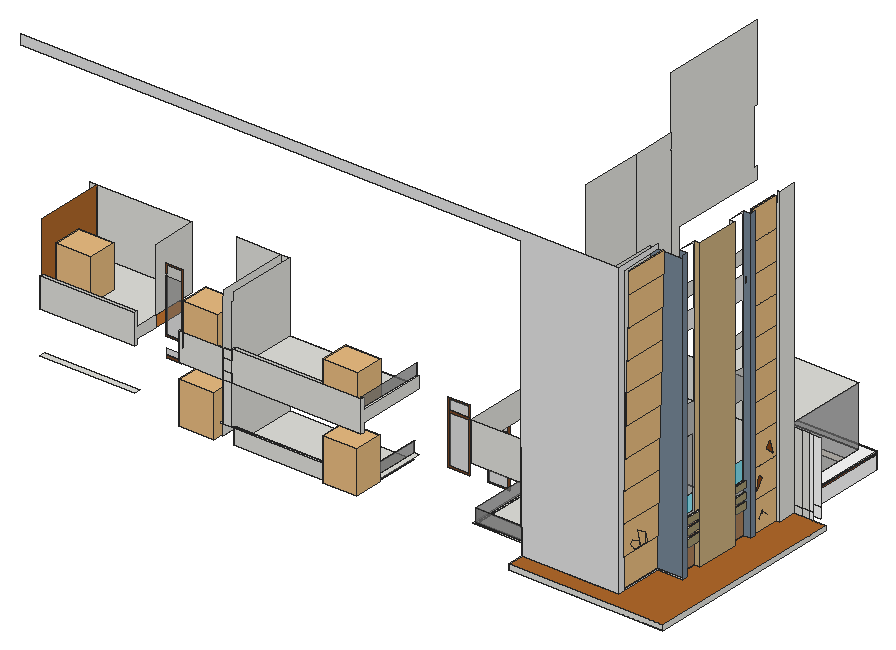
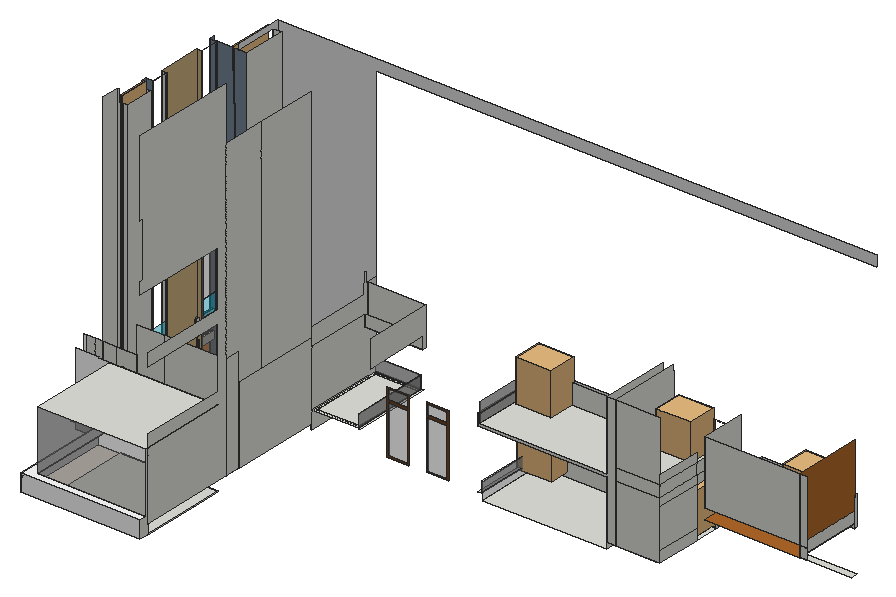
# SketchUp Ruby script. Lengths in inches.
U = 1.inch
M = Sketchup.active_model
def pt(a) = Geom::Point3d.new(a.map { |v| v * U })
def face(e, loops, mat)
  f = e.add_face(loops[0].map { |a| pt(a) })
  loops[1..].each { |l| e.add_face(l.map { |a| pt(a) }).erase! }
  f.material = f.back_material = mat if mat
  f
end
# faces: each face lists its corners as indices into pts; further lists are holes
def faces(e, pts, list, mat = nil) = list.each { |f| face(e, (f[0].is_a?(Array) ? f : [f]).map { |l| l.map { |i| pts[i] } }, mat) }
# xy, xz, yz: faces in a plane at the given z, y or x. An outline is a flat list of corners, or four numbers for a rectangle; further outlines are holes
def ring(l) = l.size == 4 ? [[l[0], l[1]], [l[2], l[1]], [l[2], l[3]], [l[0], l[3]]] : l.each_slice(2).to_a
def flat(e, list, mat, &to3) = list.each { |f| face(e, (f[0].is_a?(Array) ? f : [f]).map { |l| ring(l).map { |u, v| to3.(u, v) } }, mat) }
def xy(e, z, list, mat = nil) = flat(e, list, mat) { |x, y| [x, y, z] }
def xz(e, y, list, mat = nil) = flat(e, list, mat) { |x, z| [x, y, z] }
def yz(e, x, list, mat = nil) = flat(e, list, mat) { |y, z| [x, y, z] }
def lines(e, pts, list) = list.each { |a, b| e.add_line(pt(pts[a]), pt(pts[b])) }
# prism: a flat outline (further loops are holes) pulled along v
def prism(e, loops, v, mat = nil)
  f = face(e, loops, mat); d = Geom::Vector3d.new(v.map { |x| x * U })
  f.pushpull(f.normal.samedirection?(d) ? d.length : -d.length)
end
def box(e, o, s, mat = nil) = prism(e, [[o, [o[0] + s[0], o[1], o[2]], [o[0] + s[0], o[1] + s[1], o[2]], [o[0], o[1] + s[1], o[2]]]], [0, 0, s[2]], mat)
def at(x, y, z, deg = 0) = Geom::Transformation.translation(pt([x, y, z])) * Geom::Transformation.rotation(ORIGIN, Z_AXIS, deg.degrees)
def axes(o, x, y, z) = Geom::Transformation.new([*x, 0, *y, 0, *z, 0, *pt(o).to_a, 1])
def part(name) = M.definitions.add(name)
# library, detail: a bought-in or finely detailed component or shape, given as its bounding box
def library(name, o, s) = part(name).tap { |d| box(d.entities, o, s) }
def detail(e, o, s) = box(e.add_group.entities, o, s)
def put(e, d, t, mat = nil) = e.add_instance(d, t).tap { |i| i.material = mat if mat }
def group(e, t, mat = nil) = e.add_group.tap { |g| g.transformation = t; g.material = mat if mat }.entities
root = M.entities
M.materials.add("[0030_OldLace]").color = [253, 245, 230]
M.materials.add("[0042_Sienna]").color = [160, 82, 45]
M.materials.add("[0043_SaddleBrown]").color = [139, 69, 19]
M.materials.add("[0110_LightSlateGray]").color = [119, 136, 153]
M.materials.add("[0128_White]").color = [255, 255, 255]
M.materials.add("[0129_WhiteSmoke]").color = [245, 245, 245]
M.materials.add("[Polished Concrete Old]").color = [229, 229, 229]
M.materials.add("[Translucent Glass Gray]").color = [128, 128, 128]
M.materials["[Translucent Glass Gray]"].alpha = 0.5
M.materials.add("[Translucent Glass Tinted]").color = [8, 201, 241]
M.materials["[Translucent Glass Tinted]"].alpha = 0.48
M.materials.add("[Wood Bamboo]").color = [177, 105, 43]
M.materials.add("[Wood Floor Light]").color = [204, 176, 127]
M.materials.add("[Wood Floor]").color = [155, 105, 61]
M.materials.add("[Wood Lumber ButtJoined]").color = [164, 152, 112]
M.materials.add("[Wood Veneer 01]").color = [120, 70, 37]
c1 = library("Plant+(3)",[-15.5,2.64,0],[117.71,96.38,184.75])
c2 = library("Group\#2",[2.66,0,2.66],[81.3,1.18,61.61])
c3 = part("Decorative screen panels")
put(c3.entities,c2,axes([-6.34,-1.57,-2.66],[1.10721,0,0],[0,-0.19,0],[0,0,1]))
put(c3.entities,c2,axes([-6.34,0,59.33],[1.10721,0,0],[0,-0.19,0],[0,0,1]))
put(c3.entities,c2,axes([-6.34,1.57,121.32],[1.10721,0,0],[0,-0.19,0],[0,0,1]))
put(c3.entities,c2,axes([-6.34,3.15,183.3],[1.10721,0,0],[0,-0.19,0],[0,0,1]))
put(c3.entities,c2,axes([-6.34,4.72,245.29],[1.10721,0,0],[0,-0.19,0],[0,0,1]))
put(c3.entities,c2,axes([-6.34,6.3,307.28],[1.10721,0,0],[0,-0.19,0],[0,0,1]))
put(c3.entities,c2,axes([-6.34,7.875,369.27],[1.10721,0,0],[0,-0.19,0],[0,0,1]))
put(c3.entities,c2,axes([-6.34,9.45,431.25],[1.10721,0,0],[0,-0.19,0],[0,0,1]))
put(c3.entities,c2,axes([-6.34,11.02,493.24],[1.10721,0,0],[0,-0.19,0],[0,0,1]))
put(c3.entities,c2,axes([-6.34,10.61,555.97],[1.10721,0,0],[0,1.4896,0],[0,0,0.7225]))
put(c3.entities,c2,axes([-255.6,43,-5.47],[0.74066,0,0],[0,3.6727,0],[0,0,1]))
put(c3.entities,c2,axes([-255.6,43,55.32],[0.74066,0,0],[0,3.6727,0],[0,0,1]))
put(c3.entities,c2,axes([-255.6,43,116.1],[0.74066,0,0],[0,3.6727,0],[0,0,1]))
put(c3.entities,c2,axes([-255.6,43,176.89],[0.74066,0,0],[0,3.6727,0],[0,0,1]))
put(c3.entities,c2,axes([-255.6,43,237.68],[0.74066,0,0],[0,3.6727,0],[0,0,1]))
put(c3.entities,c2,axes([-255.6,43,298.47],[0.74066,0,0],[0,3.6727,0],[0,0,1]))
put(c3.entities,c2,axes([-255.6,43,359.26],[0.74066,0,0],[0,3.6727,0],[0,0,1]))
put(c3.entities,c2,axes([-255.6,43,420.05],[0.74066,0,0],[0,3.6727,0],[0,0,1]))
put(c3.entities,c2,axes([-255.6,43,480.84],[0.74066,0,0],[0,3.6727,0],[0,0,1]))
put(c3.entities,c2,axes([-255.6,43,543.4],[0.74066,0,0],[0,3.6727,0],[0,0,1]))
xy(root,140.13,[[1381.11,725.91,1632.4375,929.16]],"[0030_OldLace]")
xy(root,141.5625,[[1381.11,725.91,1583.5,909.71]])
xy(root,142.65,[[760.05,334.2,1021.125,480.63]])
xy(root,150.5625,[[1381.11,278.66,1429.5,313.35],[1429.5,278.66,1452.81,322.22],[1452.81,278.66,1502.3,315.91],[1502.3,278.66,1524.96,322.22],[1524.96,278.66,1576.59,313.35],
  [1576.59,278.66,1590.59,322.22],[1590.59,278.66,1641.67,315.41],[1641.67,278.66,1659.15,322.22],[1659.15,278.66,1705.61,315.28],[1524.96,313.35,1576.59,322.22],
  [1590.59,315.41,1641.67,322.22],[1452.81,315.91,1502.3,322.22],[1378.67,335.28,1381.11,480.63]])
xy(root,155.59,[[648.14,334.07,656.67,480.63],[656.67,334.07,740.81,480.63],[1023.09,334.2,1031.24,480.63]])
xy(root,161,[[1378.67,480.63,1381.11,480.63,1381.11,703.91],[1381.11,480.63,1414.17,669.54],[1414.17,480.63,1512.23,481.99],[1414.17,481.99,1512.23,669.54],[1381.11,669.54,1414.17,703.91],
  [1414.17,669.54,1512.23,701.73],[1512.23,669.54,1567.08,703.91],[1414.17,701.73,1512.23,703.91]])
xy(root,161,[[1381.11,278.66,1705.61,278.66,1705.61,703.91,1639.62,703.91,1639.62,666.21,1618,666.21,1618,606,1636.25,606,1636.25,594.34,1621.75,594.34,1621.75,558.89,1632.37,558.89,1632.37,467.07,1621.75,467.07,1621.75,427.98,1636.25,427.98,1636.25,415.98,1584.12,415.98,1584.12,313.35,1381.11,313.35],[1381.11,313.35,1414.17,480.63],[1414.17,313.35,1512.23,480.63],[1512.23,313.35,1512.23,669.54,1567.08,669.54,1567.08,703.91,1639.62,703.91,1639.62,666.21,1618,666.21,1618,606,1636.25,606,1636.25,594.34,1621.75,594.34,1621.75,558.89,1632.37,558.89,1632.37,467.07,1621.75,467.07,1621.75,427.98,1636.25,427.98,1636.25,415.98,1584.12,415.98,1584.12,313.35]],"[Wood Bamboo]")
xy(root,161.5625,[[1378.67,480.63,1512.23,669.54]])
xy(root,163.82,[[1566.87,325.97,1584.12,415.98]])
xy(root,168.48,[[1629.9375,725.91,1632.4375,929.16]])
xy(root,169.9375,[[1629.9375,725.91,1632.4375,929.16]])
xy(root,170.64,[[356.17,329.32,555.3,342.5]])
xy(root,172.02,[[1627,725.91,1632.4375,929.16]])
xy(root,173.15,[[1627,725.91,1632.4375,929.16]])
xy(root,175.875,[[1607.97,725.91,1607.97,913.9375,1381.11,913.9375,1381.11,929.16,1632.4375,929.16,1632.4375,725.91]],"[0128_White]")
xy(root,178.02,[[648.14,329.32,760.05,334.07],[760.05,329.32,1031.24,334.2],[1021.125,334.2,1023.09,480.63]])
xy(root,186.5625,[[1283.79,319.97,1374.49,474.01]])
xy(root,186.6875,[[1277.17,313.35,1381.11,313.35,1381.11,316.58,1281.11,316.58,1281.11,480.63,1277.17,480.63],[[1281.7,317.14,1378.67,480.63],[1283.79,319.97,1374.49,474.01]],[1378.67,317.14,1381.11,335.28]])
xy(root,209.76,[[1627.29,427.98,1631.48,467.73]])
xy(root,213.16,[[1623.97,558.89,1626.85,597.76]])
xy(root,214.5625,[[1378.67,313.35,1381.11,316.58],[1281.11,316.58,1378.67,316.58,1378.67,317.14,1281.7,317.14,1281.7,317.64,1281.11,317.64],[1378.67,316.58,1381.11,317.14],[1281.11,317.64,1281.7,480.63]])
xy(root,226.11,[[1627.29,427.98,1631.48,467.73]])
xy(root,226.13,[[1623.97,558.89,1626.85,597.76]])
xy(root,231.98,[[1623.97,558.89,1626.85,595.51]])
xy(root,233.59,[[1627.29,427.98,1631.48,471.48]])
xy(root,243.66,[[1623.97,558.89,1626.85,595.51]])
xy(root,246.87,[[1627.29,427.98,1631.48,471.48]])
xy(root,251.85,[[1623.97,558.89,1626.85,594.14]])
xy(root,253.24,[[1627.29,427.98,1631.48,471.48]])
xy(root,259.34,[[356.17,329.32,555.3,335.15]])
xy(root,261.04,[[648.14,329.32,760.05,331.76],[760.05,329.32,1031.24,335.17]])
xy(root,264.6,[[1623.97,558.89,1626.85,594.14]])
xy(root,266.59,[[1627.29,427.98,1631.48,471.48]])
xy(root,268.96,[[341.11,480.24,356.17,480.63]])
xy(root,268.96,[[356.17,335.15,555.3,480.63]],"[Wood Bamboo]")
xy(root,278.66,[[740.81,329.32,760.05,331.76]])
xy(root,278.66,[[648.14,331.76,740.81,481.88],[760.05,335.17,1031.24,480.63]],"[Wood Floor]")
xy(root,283.1875,[[1256.11,335.28,1378.67,342.41]])
xy(root,284.41,[[760.05,336.23,1025.87,480.63]])
xy(root,292.29,[[356.17,336.26,555.3,480.63],[341.11,480.21,356.17,480.63]])
xy(root,302.85,[[740.81,329.32,760.05,331.76],[648.14,331.76,740.81,481.88],[1026.95,336.23,1031.24,480.63]])
xy(root,303,[[1381.11,725.91,1607.97,913.9375]])
xz(root,278.66,[[1381.11,150.5625,1705.61,161]])
xz(root,313.35,[[1381.11,161,1584.12,161,1584.12,774.125,328.44,774.125,328.44,752.13,1378.67,752.13,1378.67,214.5625,1381.11,214.5625]],"[Polished Concrete Old]")
xz(root,316.58,[[1281.11,186.6875,1381.11,214.5625]],"[Translucent Glass Gray]")
xz(root,317.14,[[1281.7,186.6875,1378.67,214.5625],[1378.67,186.6875,1381.11,214.5625]],"[Translucent Glass Gray]")
xz(root,319.97,[[1283.79,186.5625,1374.49,186.6875]])
xz(root,325.97,[[1566.87,163.82,1584.12,764]])
xz(root,329.32,[[740.81,178.02,760.05,261.04],[356.17,259.34,555.3,259.34,555.3,321.06,490.96,321.16,356.17,321.16],[648.14,261.04,740.81,320.91],[740.81,261.04,760.05,278.66],[760.05,261.04,1031.24,326.04],
  [740.81,278.66,760.05,302.85],[740.81,302.85,760.05,320.91]])
xz(root,331.76,[[648.14,261.04,760.05,278.66],[648.14,302.85,760.05,320.91]])
xz(root,334.2,[[760.05,142.65,1021.125,178.02],[1023.09,155.59,1031.24,178.02]])
xz(root,335.15,[[356.17,259.34,555.3,268.96]])
xz(root,335.17,[[760.05,261.04,1031.24,278.66]])
xz(root,335.28,[[1378.67,150.5625,1381.11,186.6875],[1256.11,283.1875,1378.67,364.5625]])
xz(root,336.23,[[760.05,284.41,1025.87,326.04],[1026.95,302.85,1031.24,326.04]])
xz(root,336.26,[[356.17,292.29,555.3,321.16]])
xz(root,342.41,[[1256.11,283.1875,1378.67,307.875]])
xz(root,384.82,[[578.28,225.92,609.63,239.61],[578.02,263.16,609.9,373.61]],"[Translucent Glass Gray]")
xz(root,384.82,[[578.28,220.2,609.63,225.92],[575.9,261.04,612.02,261.04,612.02,397.85,575.9,397.85,575.9,378.89,578.02,378.89,578.02,395.73,609.9,395.73,609.9,263.16,578.02,263.16,578.02,373.61,575.9,373.61]],"[Wood Veneer 01]")
xz(root,415.98,[[1584.12,161,1636.25,163.82]])
xz(root,415.98,[[1566.87,163.82,1636.25,764]],"[0110_LightSlateGray]")
xz(root,427.98,[[[1621.75,161,1636.25,770.68],[1627.32,411.86,1631.63,468.47],[1629.07,602.14,1631.5,643.95],[1630.2,723.3125,1632.07,769.27],[1627.29,209.76,1631.48,226.11],[1627.29,253.24,1631.48,266.59],[1627.29,233.59,1631.48,246.87]]],"[0110_LightSlateGray]")
xz(root,467.07,[[1621.75,161,1632.37,161,1632.37,766.85,1632.07,766.85,1632.07,757.6,1630.2,757.6,1630.2,768.01,1632.37,768.01,1632.37,770.68,1621.75,770.68]],"[Wood Floor Light]")
xz(root,467.73,[[1627.29,209.76,1631.48,226.11]])
xz(root,471.48,[[1627.29,233.59,1631.48,246.87],[1627.29,253.24,1631.48,266.59]])
xz(root,474.01,[[1283.79,186.5625,1374.49,186.6875]])
xz(root,480.63,[[1378.67,150.5625,1381.11,161],[648.14,155.59,740.81,429.57],[740.81,155.59,760.05,155.59,760.05,278.66,1031.24,278.66,1031.24,302.85,1026.95,302.85,1026.95,326.04,1025.87,326.04,1025.87,284.41,760.05,284.41,760.05,429.57,740.81,429.57],[1378.67,161,1381.11,161.5625],[1381.11,161,1512.23,161.5625],
  [1378.67,161.5625,1381.11,322.75],[341.11,292.29,356.17,425.41],[356.17,292.29,555.3,425.41]])
xz(root,480.63,[[1177.47,156.4,1218.53,256.34],[1095.43,156.54,1136.33,256.96],[1177.47,261.53,1218.53,283.64],[1095.43,262.41,1136.33,283.51]],"[Translucent Glass Gray]")
xz(root,480.63,[[[1092.83,153.9375,1138.93,286.11],[1095.43,156.54,1136.33,283.51]],[[1175.01,153.9375,1221,286.11],[1177.47,156.4,1218.53,283.64]],[1177.47,256.34,1218.53,261.53],[1095.43,256.96,1136.33,262.41]],"[Wood Veneer 01]")
xz(root,481.88,[[648.14,278.66,740.81,302.85]])
xz(root,558.89,[[[1621.75,161,1632.37,770.68],[1625.18,417.71,1628.93,476.71],[1623.97,213.16,1626.85,264.6],[1624.9,620.41,1628.78,620.41,1628.78,649.25,1624.78,649.25,1624.78,636.65,1628.78,636.65,1628.78,630.91,1624.9,630.91],[1624.7,728.9,1626.82,768.15],[1623.49,606.8,1627.24,616.24]],[1623.97,226.13,1626.85,231.98],[1623.97,243.66,1626.85,251.85]])
xz(root,594.14,[[1623.97,251.85,1626.85,264.6]])
xz(root,594.34,[[[1621.75,161,1636.25,770.68],[1624.78,636.65,1628.78,649.25],[1624.7,728.9,1626.82,740.75]]],"[0110_LightSlateGray]")
xz(root,595.51,[[1623.97,231.98,1626.85,243.66]])
xz(root,597.76,[[1623.97,213.16,1626.85,226.13]])
xz(root,606,[[1618,161,1618,757.41,1635.25,757.41,1635.25,770.68,1636.25,770.68,1636.25,161]])
xz(root,666.21,[[1618,161,1639.62,161,1639.62,781.4375,1635.25,781.4375,1635.25,757.41,1618,757.41]])
xz(root,669.54,[[1381.11,161,1512.23,161.5625],[1512.23,161,1567.08,177.0625],[1378.67,161.5625,1381.11,322.75],[1381.11,161.5625,1381.11,322.75,1567.08,322.75,1567.08,177.0625,1512.23,177.0625,1512.23,161.5625]])
xz(root,703.91,[[1381.11,161,1512.23,379.5625],[1512.23,161,1567.08,379.5625],[1567.08,161,1611.26,177.0625],[1611.26,161,1639.62,177.0625],[1639.62,161,1655.44,177.0625],
  [1655.44,161,1672.48,177.0625],[1567.08,177.0625,1611.26,322.75],[1611.26,177.0625,1639.62,322.75],[1639.62,177.0625,1655.44,322.75],[1655.44,177.0625,1672.48,322.75]])
xz(root,703.91,[[1678.36,150.5625,1705.61,161],[1672.48,161,1678.36,177.0625],[1672.48,177.0625,1678.36,322.75]],"[0128_White]")
xz(root,725.91,[[1381.11,140.13,1583.5,141.5625],[1381.11,303,1583.5,304.04]])
xz(root,725.91,[[1632.4375,153.57,1678.36,153.57,1678.36,177.0625,1632.4375,177.0625,1632.4375,173.15,1627,173.15,1627,172.02,1632.4375,172.02,1632.4375,169.9375,1629.9375,169.9375,1629.9375,168.48,1632.4375,168.48],[1607.97,175.875,1632.4375,175.875,1632.4375,177.0625,1678.36,177.0625,1678.36,306.29,1631,306.29,1631,305.16,1632.4375,305.16,1632.4375,304.04,1583.5,304.04,1583.5,303,1607.97,303]],"[0128_White]")
xz(root,913.9375,[[1381.11,175.875,1607.97,303]],"[Translucent Glass Gray]")
xz(root,929.16,[[1381.11,140.13,1632.4375,140.13,1632.4375,168.48,1629.9375,168.48,1629.9375,169.9375,1632.4375,169.9375,1632.4375,172.02,1627,172.02,1627,173.15,1632.4375,173.15,1632.4375,175.875,1381.11,175.875]],"[0128_White]")
yz(root,356.17,[[329.32,259.34,334.16,321.16],[334.16,259.34,335.15,268.96],[334.16,268.96,334.16,321.16,336.26,321.16,336.26,292.29,480.21,292.29,480.24,268.96],[480.24,268.96,480.21,292.29,480.63,292.29,480.63,268.96],[480.21,292.29,480.02,425.41,480.63,425.41,480.63,292.29]])
yz(root,356.17,[[336.26,292.29,336.26,321.16,334.16,321.16,334.16,417.48,335.25,417.48,335.25,425.41,480.02,425.41,480.21,292.29]],"[Wood Bamboo]")
yz(root,555.3,[[329.32,259.34,335.15,259.34,335.15,268.96,384.82,268.96,384.82,292.29,336.26,292.29,336.26,321.16,329.32,321.16],[384.82,292.29,480.63,425.41]])
yz(root,648.14,[[329.32,155.59,334.07,178.02],[384.82,155.59,480.63,178.02],[384.82,178.02,480.63,261.04],[329.32,261.04,331.76,278.66],[331.76,261.04,384.82,278.66],
  [384.82,261.04,480.63,278.66],[329.32,278.66,384.82,302.85],[384.82,278.66,480.63,302.85],[480.63,278.66,481.88,302.85],[329.32,302.85,331.76,320.91],
  [384.82,302.85,480.63,320.91]])
yz(root,740.81,[[329.32,155.59,480.63,278.66],[329.32,278.66,480.63,302.85],[480.63,278.66,481.88,302.85],[329.32,302.85,329.32,417.33,330.51,417.33,330.51,429.57,480.63,429.57,480.63,302.85]])
yz(root,760.05,[[334.2,142.65,480.63,142.65,480.63,278.66,335.17,278.66,335.17,261.04,329.32,261.04,329.32,178.02,334.2,178.02],[329.32,261.04,331.76,278.66],[336.23,284.41,480.63,284.41,480.63,429.57,334.64,429.57,334.64,417.38,333.68,417.38,333.68,413.45,329.32,413.45,329.32,326.04,336.23,326.04],[329.32,302.85,331.76,320.91]])
yz(root,1021.125,[[334.2,142.65,480.63,178.02]],"[Translucent Glass Gray]")
yz(root,1023.09,[[334.2,155.59,480.63,178.02]],"[Translucent Glass Gray]")
yz(root,1025.87,[[336.23,284.41,480.63,326.04]],"[Translucent Glass Gray]")
yz(root,1026.95,[[336.23,302.85,480.63,326.04]],"[Translucent Glass Gray]")
yz(root,1031.24,[[329.32,261.04,335.17,261.04,335.17,278.66,480.63,278.66,480.63,302.85,336.23,302.85,336.23,326.04,329.32,326.04]])
yz(root,1256.11,[[335.28,283.1875,335.28,364.5625,480.63,364.5625,480.63,307.875,342.41,307.875,342.41,283.1875]])
yz(root,1281.11,[[316.58,186.6875,317.64,214.5625]])
yz(root,1281.11,[[317.64,186.6875,480.63,214.5625]],"[Translucent Glass Gray]")
yz(root,1281.7,[[317.14,186.6875,480.63,214.5625]],"[Translucent Glass Gray]")
yz(root,1283.79,[[319.97,186.5625,474.01,186.6875]])
yz(root,1374.49,[[319.97,186.5625,474.01,186.6875]])
yz(root,1378.67,[[335.28,150.5625,480.63,186.6875],[480.63,161.5625,669.54,322.75],[317.14,186.6875,317.14,214.5625,313.35,214.5625,313.35,283.1875,342.41,283.1875,342.41,307.875,480.63,307.875,480.63,186.6875],[313.35,283.1875,335.28,364.5625],[335.28,283.1875,335.28,364.5625,340.07,364.5625,340.07,385.9375,341.7,385.9375,341.7,364.5625,344.87,364.5625,344.87,344.1875,480.63,344.1875,480.63,307.875,342.41,307.875,342.41,283.1875]])
yz(root,1381.11,[[725.91,140.13,789.03,141.5625],[789.03,140.13,909.71,141.5625],[909.71,140.13,929.16,140.13,929.16,175.875,913.9375,175.875,913.9375,303,909.71,303],[278.66,150.5625,313.35,161],[335.28,150.5625,480.63,161],
  [313.35,161,335.28,186.6875],[480.63,161,611.07,784.875],[611.07,161,669.54,161,669.54,379.5625,703.91,379.5625,703.91,784.875,611.07,784.875],[669.54,161,703.91,379.5625],[703.91,161,909.71,161,909.71,303,725.91,303,725.91,304.04,909.71,304.04,909.71,328.75,725.91,328.75,725.91,456.48,909.71,456.48,909.71,482.34,725.91,482.34,725.91,598.78,929.16,598.78,929.16,624.41,922.47,624.41,922.47,738.98,929.53,738.98,929.53,897.8125,703.91,897.8125],
  [313.35,186.6875,316.58,214.5625],[316.58,186.6875,317.14,214.5625],[725.91,303,909.71,304.04]])
yz(root,1512.23,[[480.63,146.92,481.99,148.28],[480.63,161,481.99,161.5625],[481.99,161,669.54,161.5625]])
yz(root,1512.23,[[480.63,148.28,481.99,161]],"[0129_WhiteSmoke]")
yz(root,1512.23,[[669.54,148.28,701.73,161]],"[Wood Floor Light]")
yz(root,1566.87,[[325.97,163.82,415.98,764]])
yz(root,1567.08,[[669.54,161,703.91,177.0625],[669.54,177.0625,703.91,322.75]])
yz(root,1582.4,[[343.8125,182.27,362.75,198.07,349.77,208.07]],"[0043_SaddleBrown]")
yz(root,1584.12,[[313.35,161,415.98,161,415.98,163.82,325.97,163.82,325.97,764,415.98,764,415.98,774.125,313.35,774.125]],"[Polished Concrete Old]")
yz(root,1585.55,[[384.61,288.59,384.61,308.26,361.93,323.73,371.74,288.63]],"[0043_SaddleBrown]")
yz(root,1607.97,[[725.91,175.875,913.9375,303]],"[Translucent Glass Gray]")
yz(root,1618,[[606,161,666.21,757.41]])
yz(root,1621.75,[[[427.98,161,467.07,770.68],[429.83,265.5,460.95,411.3125],[433.29,471.78,463.16,609.125],[430.16,647.23,463.1,769.33]],[[558.89,161,594.34,770.68],[560.74,263.99,592.86,415.97],[561.04,477.54,592.04,604.41],[560.31,651.2,560.31,768.52,593.12,768.52,593.12,683.14,593.25,683.14,593.25,651.2]],[429.83,300.5,460.95,411.3125]],"[Translucent Glass Gray]")
yz(root,1621.75,[[560.74,263.99,592.86,303.84],[429.83,265.5,460.95,300.5]],"[Translucent Glass Tinted]")
yz(root,1623.97,[[558.89,213.16,597.76,226.13],[558.89,231.98,595.51,243.66],[558.89,251.85,594.14,264.6]])
yz(root,1626.85,[[558.89,213.16,597.76,226.13],[558.89,231.98,595.51,243.66],[558.89,251.85,594.14,264.6]],"[Wood Lumber ButtJoined]")
yz(root,1627,[[725.91,172.02,929.16,173.15]])
yz(root,1627.29,[[427.98,209.76,467.73,226.11],[427.98,233.59,471.48,246.87],[427.98,253.24,471.48,266.59]])
yz(root,1629.9375,[[725.91,168.48,929.16,169.9375]])
yz(root,1631.46,[[616.3,237.86,630.61,256.04,621.92,266.05],[659.78,290.25,650.3,317.64,639.82,308.53]],"[0043_SaddleBrown]")
yz(root,1631.48,[[427.98,209.76,467.73,226.11],[427.98,233.59,471.48,246.87],[427.98,253.24,471.48,266.59]],"[Wood Lumber ButtJoined]")
yz(root,1632.37,[[467.07,161,558.89,770.68]],"[Wood Floor Light]")
yz(root,1632.4375,[[725.91,175.2,929.16,175.875]])
yz(root,1632.4375,[[725.91,169.9375,929.16,172.02],[725.91,173.15,929.16,175.2]],"[0042_Sienna]")
yz(root,1632.4375,[[725.91,140.13,929.16,168.48]],"[0128_White]")
yz(root,1636.25,[[415.98,161,427.98,770.68],[594.34,161,606,770.68]],"[0110_LightSlateGray]")
yz(root,1639.62,[[666.21,161,703.91,781.4375]])
yz(root,1705.61,[[278.66,150.5625,703.91,161]])
p = [[1583.97,389.48,226.61],[1583.9,413.33,226.61],[1583.97,384.61,246.27],[356.17,480.24,268.96],[356.17,480.21,292.29],[341.11,480.21,292.29],
  [341.11,480.24,268.96],[656.67,334.07,155.59],[656.67,329.32,155.59],[1583.97,370.97,225.8],[1583.97,362.75,260.05],[1583.9,384.61,246.27],
  [1583.9,384.61,226.64],[1583.9,369.87,226.63],[1583.97,355.59,226.63],[1583.97,343.4,241.42],[1583.9,349.31,247.125],[1583.97,367.64,237.13],
  [1630.01,635.37,161.82],[1630.54,633.43,174.65],[1631.46,630.06,196.94],[1631.46,643.74,182.95],[1618,655.91,161],[1630.01,632.08,184.9],
  [1631.46,622.5,183.56],[1631.46,621.05,183.95]]
faces(root,p,[[0,1,2]],"[0043_SaddleBrown]")
faces(root,p,[[3,4,5,6]])
lines(root,p,[[7,8],[9,10],[10,11],[11,12],[12,9],[0,11],[13,0],[14,15],[15,16],[16,17],[17,13],[13,14],
  [18,19],[20,21],[21,22],[22,18],[23,20],[24,20],[19,20],[25,19]])
put(root,c1,axes([970.875,313.35,151.28],[0.62,0,0],[0,0.62,0],[0,0,0.4774]))
put(root,c1,axes([669.125,313.35,151.28],[0.62,0,0],[0,0.62,0],[0,0,0.4774]))
put(root,c3,at(1584.12,412.58,163.82,-90),"[0043_SaddleBrown]")
put(root,c1,axes([959.125,329.32,283.68],[0.62,0,0],[0,0.62,0],[0,0,0.4774]))
put(root,c1,axes([665.58,329.32,290.19],[0.62,0,0],[0,0.62,0],[0,0,0.4774]))
put(root,c1,axes([384.34,347.69,292.29],[0.62,0,0],[0,0.62,0],[0,0,0.4774]))
